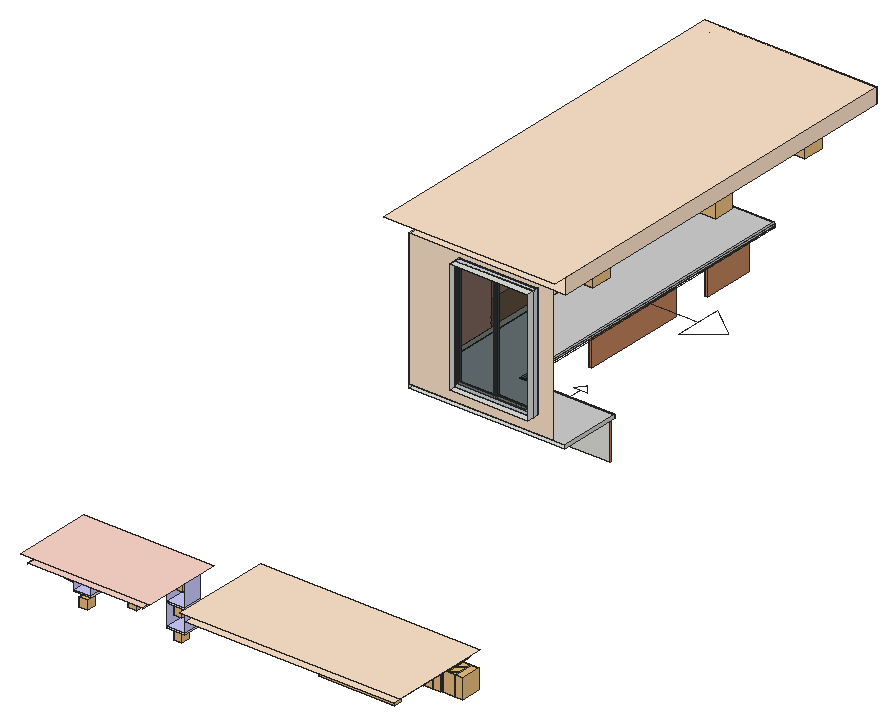
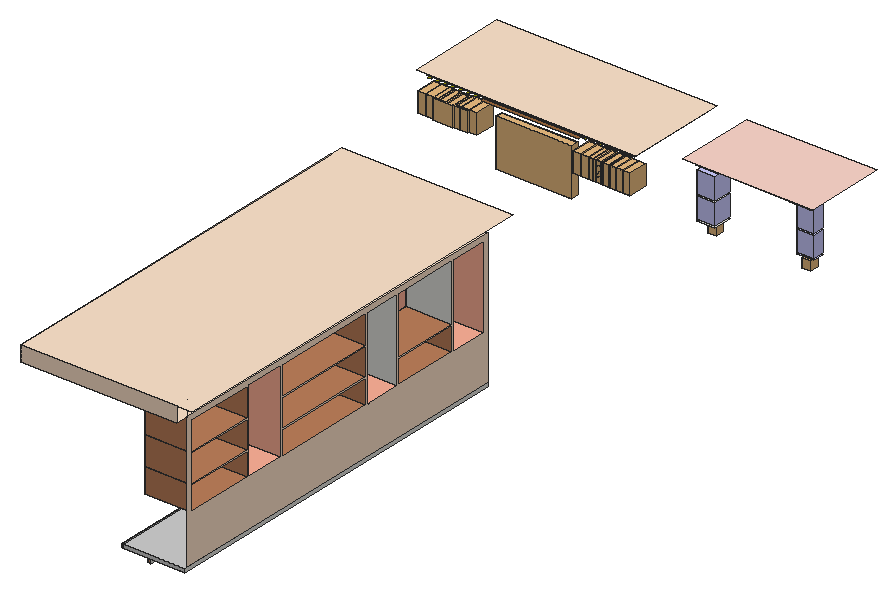
# SketchUp Ruby script. Lengths in inches.
U = 1.inch
M = Sketchup.active_model
def pt(a) = Geom::Point3d.new(a.map { |v| v * U })
def face(e, loops, mat)
  f = e.add_face(loops[0].map { |a| pt(a) })
  loops[1..].each { |l| e.add_face(l.map { |a| pt(a) }).erase! }
  f.material = f.back_material = mat if mat
  f
end
# faces: each face lists its corners as indices into pts; further lists are holes
def faces(e, pts, list, mat = nil) = list.each { |f| face(e, (f[0].is_a?(Array) ? f : [f]).map { |l| l.map { |i| pts[i] } }, mat) }
# xy, xz, yz: faces in a plane at the given z, y or x. An outline is a flat list of corners, or four numbers for a rectangle; further outlines are holes
def ring(l) = l.size == 4 ? [[l[0], l[1]], [l[2], l[1]], [l[2], l[3]], [l[0], l[3]]] : l.each_slice(2).to_a
def flat(e, list, mat, &to3) = list.each { |f| face(e, (f[0].is_a?(Array) ? f : [f]).map { |l| ring(l).map { |u, v| to3.(u, v) } }, mat) }
def xy(e, z, list, mat = nil) = flat(e, list, mat) { |x, y| [x, y, z] }
def xz(e, y, list, mat = nil) = flat(e, list, mat) { |x, z| [x, y, z] }
def yz(e, x, list, mat = nil) = flat(e, list, mat) { |y, z| [x, y, z] }
def lines(e, pts, list) = list.each { |a, b| e.add_line(pt(pts[a]), pt(pts[b])) }
# prism: a flat outline (further loops are holes) pulled along v
def prism(e, loops, v, mat = nil)
  f = face(e, loops, mat); d = Geom::Vector3d.new(v.map { |x| x * U })
  f.pushpull(f.normal.samedirection?(d) ? d.length : -d.length)
end
def box(e, o, s, mat = nil) = prism(e, [[o, [o[0] + s[0], o[1], o[2]], [o[0] + s[0], o[1] + s[1], o[2]], [o[0], o[1] + s[1], o[2]]]], [0, 0, s[2]], mat)
def at(x, y, z, deg = 0) = Geom::Transformation.translation(pt([x, y, z])) * Geom::Transformation.rotation(ORIGIN, Z_AXIS, deg.degrees)
def axes(o, x, y, z) = Geom::Transformation.new([*x, 0, *y, 0, *z, 0, *pt(o).to_a, 1])
def part(name) = M.definitions.add(name)
# library, detail: a bought-in or finely detailed component or shape, given as its bounding box
def library(name, o, s) = part(name).tap { |d| box(d.entities, o, s) }
def detail(e, o, s) = box(e.add_group.entities, o, s)
def put(e, d, t, mat = nil) = e.add_instance(d, t).tap { |i| i.material = mat if mat }
def group(e, t, mat = nil) = e.add_group.tap { |g| g.transformation = t; g.material = mat if mat }.entities
root = M.entities
M.materials.add("[Carrera Marble]").color = [207, 207, 207]
M.materials.add("[Color B01]").color = [255, 216, 204]
M.materials.add("[Color B02]").color = [255, 178, 153]
M.materials.add("[Color C01]").color = [255, 229, 204]
M.materials.add("[Color E07]").color = [153, 153, 0]
M.materials.add("[Color F02]").color = [204, 255, 153]
M.materials.add("[Color I01]").color = [204, 204, 255]
M.materials.add("[Metal Aluminum Anodized]").color = [202, 209, 219]
M.materials.add("[Metal Seamed]").color = [118, 119, 115]
M.materials.add("[Translucent Glass Tinted]").color = [1, 25, 30]
M.materials["[Translucent Glass Tinted]"].alpha = 0.31
M.materials.add("[Wood Floor]").color = [155, 105, 61]
M.materials.add("[Wood Veneer 02]").color = [190, 128, 91]
c1 = library("Spot Light\#1",[-5.1,-5.1,-11.05],[10.2,10.2,11.05])
c2 = library("Flat screen display",[0,1.41,1.14],[35.92,0.28,20.21])
c3 = library("Spot Light\#2",[-5.1,-5.1,-11.05],[10.2,10.2,11.05])
c4 = library("Omni Light",[-12,-12,-12],[24,24,24])
c5 = part("Group33\#1")
p = [[0,0,0],[0,0,-18.23],[-8.72,0,-18.23],[56.77,-2.25,0],[-56.77,-2.25,0],[56.77,2.25,0],
  [56.77,0,0],[-56.77,2.25,0],[8.72,0,-18.23],[-56.77,0,0],[0,0,-29.51]]
lines(c5.entities,p,[[0,1],[1,2],[3,4],[5,6],[7,5],[1,8],[9,0],[0,6],[8,10],[4,9],[6,3],[2,10],
  [9,7]])
c6 = part("Rectangle Light")
put(c6.entities,c5,at(0,0,0))
c7 = part("Group35\#1")
p = [[0,0,0],[0,0,-59.7],[-29.34,0,-59.7],[191.03,-2.25,0],[-191.03,-2.25,0],[191.03,2.25,0],
  [191.03,0,0],[-191.03,2.25,0],[29.34,0,-59.7],[-191.03,0,0],[0,0,-96.64]]
lines(c7.entities,p,[[0,1],[1,2],[3,4],[5,6],[7,5],[1,8],[9,0],[0,6],[8,10],[4,9],[6,3],[2,10],
  [9,7]])
c8 = part("Rectangle Light\#1")
put(c8.entities,c7,at(0,0,0))
c9 = library("Spot Light\#3",[-5.1,-5.1,-11.05],[10.2,10.2,11.05])
c10 = part("Group\#106")
prism(c10.entities,[[[0.375,0,0],[0.375,0,57],[0.375,26.94,57],[0.375,26.94,0]],[[0.375,25.82,55.875],[0.375,1.125,55.875],[0.375,1.125,1.125],[0.375,25.82,1.125]]],[1.5,0,0])
c11 = part("Group\#67")
box(c11.entities,[0,-23.19,0],[1.125,24.69,54.75])
c12 = part("Aluminium+Channel+Glass+Window")
g1 = group(c12.entities,at(536.45,-8.32,338.57,90))
g2 = group(g1,at(73.57,-163.55,-184.94),"[Metal Aluminum Anodized]")
prism(g2,[[[0,0,136.125],[0,94.5,136.125],[0,94.5,0],[0,0,0]],[[0,2.49,3.4],[0,92.01,3.4],[0,92.01,132.72],[0,2.49,132.72]]],[5.375,0,0])
g3 = group(g1,at(76.3,-161.06,-181.54))
put(g3,c10,axes([-0.55,0,0],[1.45782,0,0],[0,1.69662,0],[0,0,2.26875]),"[Metal Seamed]")
put(g3,c11,axes([0.27,41.26,2.55],[1.45782,0,0],[0,1.69662,0],[0,0,2.26875]),"[Translucent Glass Tinted]")
g4 = group(g1,at(74.11,-117.25,-181.54))
put(g4,c10,axes([-0.55,0,0],[1.45782,0,0],[0,1.69662,0],[0,0,2.26875]),"[Metal Seamed]")
put(g4,c11,axes([0.27,41.26,2.55],[1.45782,0,0],[0,1.69662,0],[0,0,2.26875]),"[Translucent Glass Tinted]")
c13 = library("Spot Light",[-5.1,-5.1,-11.05],[10.2,10.2,11.05])
xy(root,81.2,[[164.74,586.56,240.3,588.31]])
xy(root,89.47,[[122.73,67.26,144.4375,90.2]])
xy(root,89.48,[[11.17,67.26,31.62,80.32]],"[Color I01]")
xy(root,91.47,[[122.73,67.26,144.4375,90.2]],"[Color I01]")
xy(root,91.48,[[11.17,67.26,31.62,80.32]],"[Color I01]")
xy(root,96.13,[[126.97,696.29,126.78,823.17,130.96,823.18,131.14,696.3],[126.97,871.55,126.78,932.72,130.58,932.73,130.76,871.56]])
xy(root,116.16,[[122.73,67.26,144.4375,90.2]])
xy(root,116.18,[[11.17,67.26,31.62,80.32]],"[Color I01]")
xy(root,118.16,[[122.73,67.26,144.4375,90.2]],"[Color I01]")
xy(root,118.18,[[11.17,67.26,31.62,80.32]],"[Color I01]")
xy(root,120.1875,[[207.4,109.94,211.04,115.88],[216.41,109.94,220.05,115.88],[225.42,109.94,229.06,115.88],[234.43,109.94,238.08,115.88],[243.44,109.94,247.09,115.88],
  [252.45,109.94,256.1,115.88],[392.64,109.94,396.28,115.88],[401.81,109.94,405.45,115.88],[410.97,109.94,414.62,115.88],[420.14,109.94,423.78,115.88],
  [429.31,109.94,432.95,115.88],[438.47,109.94,442.12,115.88]],"[Color F02]")
xy(root,127.26,[[164.74,586.56,240.3,588.31],[126.97,696.29,131.14,696.3,130.96,823.18,126.78,823.17],[126.97,871.55,130.76,871.56,130.58,932.73,126.78,932.72]],"[Wood Veneer 02]")
xy(root,128.0625,[[55.53,515.38,55.53,971,130.28,971,130.28,588.93,243.82,588.93,243.82,515.38]])
xy(root,132.5625,[[55.53,515.38,243.82,515.38,243.82,588.93,130.28,588.93,130.28,971,55.53,971]],"[Carrera Marble]")
xy(root,144.85,[[122.73,67.26,144.4375,90.2]],"[Color I01]")
xy(root,144.88,[[11.17,67.26,31.62,80.32]],"[Color I01]")
xy(root,147.04,[[264.93,112.26,382.43,115.88]],"[Wood Floor]")
xy(root,147.5625,[[8.49,67.26,34.3,87.7],[120.02,67.26,147.15,87.7]],"[Color I01]")
xy(root,148.5,[[[8.49,0,147.15,87.7],[46.53,12.51,48.28,12.74,49.91,13.41,51.31,14.48,52.38,15.88,53.05,17.51,53.28,19.26,53.05,21,52.38,22.63,51.31,24.03,49.91,25.1,48.28,25.78,46.53,26.01,44.79,25.78,43.16,25.1,41.76,24.03,40.6875,22.63,40.01,21,39.78,19.26,40.01,17.51,40.6875,15.88,41.76,14.48,43.16,13.41,44.79,12.74],[90.51,47.29,91.79,47.46,92.98,47.95,94,48.74,94.79,49.76,95.28,50.95,95.45,52.23,95.28,53.51,94.79,54.7,94,55.72,92.98,56.51,91.79,57,90.51,57.17,89.23,57,88.04,56.51,87.02,55.72,86.23,54.7,85.74,53.51,85.57,52.23,85.74,50.95,86.23,49.76,87.02,48.74,88.04,47.95,89.23,47.46],[126.44,11.29,127.7,11.46,128.88,11.94,129.89,12.72,130.66,13.73,131.15,14.9,131.32,16.17,131.15,17.43,130.66,18.6,129.89,19.61,128.88,20.39,127.7,20.875,126.44,21.04,125.18,20.875,124,20.39,122.99,19.61,122.22,18.6,121.73,17.43,121.57,16.17,121.73,14.9,122.22,13.73,122.99,12.72,124,11.94,125.18,11.46]],[[126.44,11.29,125.18,11.46,124,11.94,122.99,12.72,122.22,13.73,121.73,14.9,121.57,16.17,121.73,17.43,122.22,18.6,122.99,19.61,124,20.39,125.18,20.875,126.44,21.04,127.7,20.875,128.88,20.39,129.89,19.61,130.66,18.6,131.15,17.43,131.32,16.17,131.15,14.9,130.66,13.73,129.89,12.72,128.88,11.94,127.7,11.46],[126.44,12.49,127.39,12.61,128.28,12.98,129.04,13.5625,129.63,14.33,130,15.21,130.12,16.17,130,17.12,129.63,18.01,129.04,18.77,128.28,19.35,127.39,19.72,126.44,19.85,125.49,19.72,124.6,19.35,123.84,18.77,123.25,18.01,122.89,17.12,122.76,16.17,122.89,15.21,123.25,14.33,123.84,13.5625,124.6,12.98,125.49,12.61]],[[46.53,12.51,44.79,12.74,43.16,13.41,41.76,14.48,40.6875,15.88,40.01,17.51,39.78,19.26,40.01,21,40.6875,22.63,41.76,24.03,43.16,25.1,44.79,25.78,46.53,26.01,48.28,25.78,49.91,25.1,51.31,24.03,52.38,22.63,53.05,21,53.28,19.26,53.05,17.51,52.38,15.88,51.31,14.48,49.91,13.41,48.28,12.74],[46.53,15.02,47.63,15.16,48.65,15.59,49.53,16.26,50.2,17.14,50.63,18.16,50.77,19.26,50.63,20.35,50.2,21.375,49.53,22.25,48.65,22.93,47.63,23.35,46.53,23.5,45.4375,23.35,44.41,22.93,43.54,22.25,42.86,21.375,42.44,20.35,42.3,19.26,42.44,18.16,42.86,17.14,43.54,16.26,44.41,15.59,45.4375,15.16]],[[90.51,47.29,89.23,47.46,88.04,47.95,87.02,48.74,86.23,49.76,85.74,50.95,85.57,52.23,85.74,53.51,86.23,54.7,87.02,55.72,88.04,56.51,89.23,57,90.51,57.17,91.79,57,92.98,56.51,94,55.72,94.79,54.7,95.28,53.51,95.45,52.23,95.28,50.95,94.79,49.76,94,48.74,92.98,47.95,91.79,47.46],[90.51,48.76,91.41,48.88,92.24,49.22,92.96,49.78,93.52,50.49,93.86,51.33,93.98,52.23,93.86,53.13,93.52,53.97,92.96,54.68,92.24,55.24,91.41,55.58,90.51,55.7,89.61,55.58,88.77,55.24,88.05,54.68,87.5,53.97,87.16,53.13,87.04,52.23,87.16,51.33,87.5,50.49,88.05,49.78,88.77,49.22,89.61,48.88]]],"[Color B01]")
xy(root,149,[[202.89,109.94,206.54,115.88],[211.9,109.94,215.55,115.88],[220.91,109.94,224.56,115.88],[229.92,109.94,233.57,115.88],[238.94,109.94,242.58,115.88],
  [247.95,109.94,251.59,115.88],[256.96,109.94,260.6,115.88],[388.06,109.94,391.7,115.88],[397.22,109.94,400.87,115.88],[406.39,109.94,410.03,115.88],
  [415.56,109.94,419.2,115.88],[424.72,109.94,428.37,115.88],[433.89,109.94,437.53,115.88],[443.06,109.94,446.7,115.88]],"[Color E07]")
xy(root,149.6875,[[126.44,12.49,125.49,12.61,124.6,12.98,123.84,13.5625,123.25,14.33,122.89,15.21,122.76,16.17,122.89,17.12,123.25,18.01,123.84,18.77,124.6,19.35,125.49,19.72,126.44,19.85,127.39,19.72,128.28,19.35,129.04,18.77,129.63,18.01,130,17.12,130.12,16.17,130,15.21,129.63,14.33,129.04,13.5625,128.28,12.98,127.39,12.61]],"[Color B01]")
xy(root,149.8125,[[46.53,15.02,45.4375,15.16,44.41,15.59,43.54,16.26,42.86,17.14,42.44,18.16,42.3,19.26,42.44,20.35,42.86,21.375,43.54,22.25,44.41,22.93,45.4375,23.35,46.53,23.5,47.63,23.35,48.65,22.93,49.53,22.25,50.2,21.375,50.63,20.35,50.77,19.26,50.63,18.16,50.2,17.14,49.53,16.26,48.65,15.59,47.63,15.16]],"[Color B01]")
xy(root,150.875,[[90.51,48.76,89.61,48.88,88.77,49.22,88.05,49.78,87.5,50.49,87.16,51.33,87.04,52.23,87.16,53.13,87.5,53.97,88.05,54.68,88.77,55.24,89.61,55.58,90.51,55.7,91.41,55.58,92.24,55.24,92.96,54.68,93.52,53.97,93.86,53.13,93.98,52.23,93.86,51.33,93.52,50.49,92.96,49.78,92.24,49.22,91.41,48.88]],"[Color B01]")
xy(root,151.1875,[[197.89,1.64,448.06,115.88]],"[Color C01]")
xy(root,153.625,[[116.72,499.97,211.22,515.38]])
xy(root,155.125,[[0,0,156.26,96.1875]],"[Color B01]")
xy(root,158,[[190.88,1.64,455.07,122.89]],"[Color C01]")
xy(root,189.5,[[55.53,521.38,111.53,568.07],[55.53,651.49,111.53,697.87],[55.53,826.92,111.53,875.98]],"[Color B02]")
xy(root,189.5,[[55.53,568.97,111.53,650.59],[55.53,698.77,111.53,826.02],[55.53,876.88,111.53,961.6875]],"[Wood Veneer 02]")
xy(root,218.3125,[[55.53,568.97,111.53,650.59],[55.53,698.77,111.53,826.02],[55.53,876.88,111.53,961.6875]],"[Wood Veneer 02]")
xy(root,219.11,[[55.53,568.97,111.53,650.59],[55.53,698.77,111.53,826.02],[55.53,876.88,111.53,961.6875]],"[Wood Veneer 02]")
xy(root,252.6875,[[55.53,698.77,111.53,826.02],[55.53,876.88,111.53,961.6875]],"[Wood Veneer 02]")
xy(root,253.59,[[55.53,698.77,111.53,826.02],[55.53,876.88,111.53,961.6875]],"[Wood Veneer 02]")
xy(root,288.5,[[55.53,521.38,111.53,568.07],[55.53,568.97,111.53,650.59],[55.53,651.49,111.53,697.87],[55.53,826.92,111.53,875.98]],"[Color B02]")
xy(root,288.5,[[55.53,698.77,111.53,826.02],[55.53,876.88,111.53,961.6875]],"[Wood Veneer 02]")
xy(root,289.75,[[116.72,499.97,211.22,515.38]])
xy(root,294.5,[[[55.53,515.38,244.12,983.1],[215.11,894.45,218.83,895.12,222.26,896.74,225.15,899.18,227.31,902.29,228.59,905.85,228.9,909.625,228.23,913.35,226.62,916.77,224.17,919.66,221.0625,921.82,217.5,923.1,213.73,923.42,210,922.75,206.58,921.13,203.6875,918.6875,201.53,915.58,200.25,912.02,199.93,908.24,200.61,904.52,202.22,901.1,204.66,898.21,207.77,896.05,211.34,894.77],[210.38,581.74,214.09,582.23,217.54,583.66,220.5,585.93,222.78,588.89,224.21,592.35,224.69,596.05,224.21,599.75,222.78,603.21,220.5,606.17,217.54,608.45,214.09,609.875,210.38,610.36,206.68,609.875,203.23,608.45,200.26,606.17,197.99,603.21,196.56,599.75,196.07,596.05,196.56,592.35,197.99,588.89,200.26,585.93,203.23,583.66,206.68,582.23],[216.58,753.94,220.08,754.58,223.29,756.1,226.01,758.39,228.03,761.32,229.23,764.67,229.52,768.21,228.89,771.71,227.37,774.93,225.07,777.64,222.15,779.67,218.8,780.87,215.26,781.16,211.76,780.53,208.54,779.01,205.83,776.71,203.8,773.78,202.6,770.4375,202.31,766.89,202.94,763.39,204.46,760.18,206.76,757.46,209.68,755.44,213.03,754.23]],[[210.38,581.74,206.68,582.23,203.23,583.66,200.26,585.93,197.99,588.89,196.56,592.35,196.07,596.05,196.56,599.75,197.99,603.21,200.26,606.17,203.23,608.45,206.68,609.875,210.38,610.36,214.09,609.875,217.54,608.45,220.5,606.17,222.78,603.21,224.21,599.75,224.69,596.05,224.21,592.35,222.78,588.89,220.5,585.93,217.54,583.66,214.09,582.23],[210.15,583.74,213.35,584.1,216.34,585.27,218.92,587.18,220.93,589.7,222.21,592.64,222.69,595.82,222.33,599.01,221.16,602.01,219.25,604.59,216.74,606.6,213.79,607.88,210.61,608.36,207.42,608,204.43,606.83,201.84,604.92,199.84,602.41,198.55,599.46,198.07,596.28,198.43,593.09,199.61,590.09,201.51,587.51,204.03,585.5,206.97,584.22]],[[216.58,753.94,213.03,754.23,209.68,755.44,206.76,757.46,204.46,760.18,202.94,763.39,202.31,766.89,202.6,770.4375,203.8,773.78,205.83,776.71,208.54,779.01,211.76,780.53,215.26,781.16,218.8,780.87,222.15,779.67,225.07,777.64,227.37,774.93,228.89,771.71,229.52,768.21,229.23,764.67,228.03,761.32,226.01,758.39,223.29,756.1,220.08,754.58],[214.42,756.02,217.46,756.03,220.39,756.82,223.01,758.34,225.15,760.49,226.67,763.125,227.44,766.06,227.4375,769.09,226.65,772.02,225.125,774.65,222.97,776.79,220.34,778.3,217.41,779.08,214.375,779.07,211.44,778.28,208.82,776.76,206.68,774.61,205.17,771.98,204.39,769.04,204.39,766.01,205.19,763.08,206.71,760.45,208.86,758.3125,211.49,756.8]],[[215.11,894.45,211.34,894.77,207.77,896.05,204.66,898.21,202.22,901.1,200.61,904.52,199.93,908.24,200.25,912.02,201.53,915.58,203.6875,918.6875,206.58,921.13,210,922.75,213.73,923.42,217.5,923.1,221.0625,921.82,224.17,919.66,226.62,916.77,228.23,913.35,228.9,909.625,228.59,905.85,227.31,902.29,225.15,899.18,222.26,896.74,218.83,895.12],[214.42,896.85,217.55,897.26,220.46,898.47,222.96,900.39,224.88,902.89,226.09,905.81,226.5,908.93,226.09,912.0625,224.88,914.98,222.96,917.48,220.46,919.4,217.55,920.61,214.42,921.02,211.29,920.61,208.375,919.4,205.87,917.48,203.95,914.98,202.74,912.0625,202.33,908.93,202.74,905.81,203.95,902.89,205.87,900.39,208.375,898.47,211.29,897.26]]],"[Color C01]")
xy(root,296.75,[[214.42,756.02,211.49,756.8,208.86,758.3125,206.71,760.45,205.19,763.08,204.39,766.01,204.39,769.04,205.17,771.98,206.68,774.61,208.82,776.76,211.44,778.28,214.375,779.07,217.41,779.08,220.34,778.3,222.97,776.79,225.125,774.65,226.65,772.02,227.4375,769.09,227.44,766.06,226.67,763.125,225.15,760.49,223.01,758.34,220.39,756.82,217.46,756.03]],"[Color C01]")
xy(root,297.3125,[[210.15,583.74,206.97,584.22,204.03,585.5,201.51,587.51,199.61,590.09,198.43,593.09,198.07,596.28,198.55,599.46,199.84,602.41,201.84,604.92,204.43,606.83,207.42,608,210.61,608.36,213.79,607.88,216.74,606.6,219.25,604.59,221.16,602.01,222.33,599.01,222.69,595.82,222.21,592.64,220.93,589.7,218.92,587.18,216.34,585.27,213.35,584.1]],"[Color C01]")
xy(root,297.4375,[[214.42,896.85,211.29,897.26,208.375,898.47,205.87,900.39,203.95,902.89,202.74,905.81,202.33,908.93,202.74,912.0625,203.95,914.98,205.87,917.48,208.375,919.4,211.29,920.61,214.42,921.02,217.55,920.61,220.46,919.4,222.96,917.48,224.88,914.98,226.09,912.0625,226.5,908.93,226.09,905.81,224.88,902.89,222.96,900.39,220.46,898.47,217.55,897.26]],"[Color C01]")
xy(root,313,[[38.18,499.97,244.12,983.1]],"[Color C01]")
xz(root,80.32,[[11.17,91.48,31.62,116.18],[11.17,118.18,31.62,144.88]],"[Color I01]")
xz(root,87.7,[[8.49,147.5625,34.3,148.5],[120.02,147.5625,147.15,148.5]],"[Color B01]")
xz(root,90.2,[[122.73,91.47,144.4375,116.16],[122.73,118.16,144.4375,144.85]],"[Color I01]")
xz(root,515.38,[[[55.53,132.5625,228.71,294.5],[116.72,153.625,211.22,289.75]]],"[Color C01]")
xz(root,521.38,[[55.53,189.5,111.53,288.5]],"[Color B02]")
xz(root,568.07,[[55.53,189.5,111.53,288.5]],"[Color B02]")
xz(root,568.97,[[55.53,219.11,111.53,288.5]])
xz(root,568.97,[[55.53,189.5,111.53,218.3125]],"[Wood Veneer 02]")
xz(root,586.56,[[164.74,81.2,240.3,127.26]])
xz(root,588.31,[[164.74,81.2,240.3,127.26]],"[Wood Veneer 02]")
xz(root,588.93,[[130.28,128.0625,243.82,132.5625]],"[Carrera Marble]")
xz(root,650.59,[[55.53,219.11,111.53,288.5]],"[Color B02]")
xz(root,650.59,[[55.53,189.5,111.53,218.3125]],"[Wood Veneer 02]")
xz(root,651.49,[[55.53,189.5,111.53,288.5]])
xz(root,697.87,[[55.53,189.5,111.53,288.5]],"[Color B02]")
xz(root,698.77,[[55.53,189.5,111.53,218.3125],[55.53,219.11,111.53,252.6875],[55.53,253.59,111.53,288.5]],"[Wood Veneer 02]")
xz(root,826.02,[[55.53,189.5,111.53,218.3125],[55.53,219.11,111.53,252.6875],[55.53,253.59,111.53,288.5]],"[Wood Veneer 02]")
xz(root,826.92,[[55.53,189.5,111.53,288.5]],"[Color B02]")
xz(root,875.98,[[55.53,189.5,111.53,288.5]],"[Color B02]")
xz(root,876.88,[[55.53,189.5,111.53,218.3125],[55.53,219.11,111.53,252.6875],[55.53,253.59,111.53,288.5]],"[Wood Veneer 02]")
xz(root,961.6875,[[55.53,189.5,111.53,218.3125],[55.53,219.11,111.53,252.6875],[55.53,253.59,111.53,288.5]],"[Wood Veneer 02]")
xz(root,971,[[55.53,128.0625,130.28,132.5625]],"[Carrera Marble]")
xz(root,983.1,[[55.53,294.5,244.12,313]],"[Color C01]")
yz(root,8.49,[[0,147.5625,87.7,148.5]],"[Color B01]")
yz(root,11.17,[[67.26,91.48,80.32,116.18],[67.26,118.18,80.32,144.88]],"[Color I01]")
yz(root,31.62,[[67.26,89.48,80.32,91.48],[67.26,116.18,80.32,118.18]])
yz(root,31.62,[[67.26,91.48,80.32,116.18],[67.26,118.18,80.32,144.88]],"[Color I01]")
yz(root,55.53,[[515.38,128.0625,971,132.5625]])
yz(root,55.53,[[[515.38,132.5625,967.6875,294.5],[568.97,219.11,650.59,288.5],[826.92,189.5,875.98,288.5],[521.38,189.5,568.07,288.5],[651.49,189.5,697.87,288.5],[698.77,253.59,826.02,288.5],[698.77,219.11,826.02,252.6875],[698.77,189.5,826.02,218.3125],[876.88,253.59,961.6875,288.5],[876.88,219.11,961.6875,252.6875],[876.88,189.5,961.6875,218.3125],[568.97,189.5,650.59,218.3125]]],"[Color C01]")
yz(root,111.53,[[521.38,189.5,568.07,288.5],[651.49,189.5,697.87,288.5],[826.92,189.5,875.98,288.5],[568.97,219.11,650.59,288.5]],"[Color B02]")
yz(root,111.53,[[568.97,189.5,650.59,218.3125],[698.77,189.5,826.02,218.3125],[876.88,189.5,961.6875,218.3125],[698.77,219.11,826.02,252.6875],[876.88,219.11,961.6875,252.6875],
  [698.77,253.59,826.02,288.5],[876.88,253.59,961.6875,288.5]],"[Wood Veneer 02]")
yz(root,116.72,[[499.97,153.625,515.38,289.75]])
yz(root,122.73,[[67.26,91.47,90.2,116.16],[67.26,118.16,90.2,144.85]],"[Color I01]")
yz(root,130.28,[[588.93,128.0625,971,132.5625]],"[Carrera Marble]")
yz(root,144.4375,[[67.26,89.47,90.2,91.47],[67.26,116.16,90.2,118.16]])
yz(root,144.4375,[[67.26,91.47,90.2,116.16],[67.26,118.16,90.2,144.85]],"[Color I01]")
yz(root,147.15,[[0,147.5625,87.7,148.5]],"[Color B01]")
yz(root,164.74,[[586.56,81.2,588.31,127.26]])
yz(root,204.39,[[766.01,294.5,769.04,296.75]],"[Color C01]")
yz(root,211.22,[[499.97,153.625,515.38,289.75]])
yz(root,240.3,[[586.56,81.2,588.31,127.26]],"[Wood Veneer 02]")
yz(root,243.82,[[515.38,128.0625,588.93,132.5625]],"[Carrera Marble]")
yz(root,244.12,[[515.38,294.5,983.1,313]],"[Color C01]")
p = [[126.97,696.29,96.13],[126.97,696.29,127.26],[126.78,823.17,127.26],[126.78,823.17,96.13],[131.14,696.3,96.13],[131.14,696.3,127.26],
  [130.96,823.18,96.13],[130.96,823.18,127.26],[126.97,871.55,96.13],[126.97,871.55,127.26],[126.78,932.72,127.26],[126.78,932.72,96.13],
  [130.76,871.56,96.13],[130.76,871.56,127.26],[130.58,932.73,96.13],[130.58,932.73,127.26],[126.44,12.49,148.5],[125.49,12.61,148.5],
  [125.49,12.61,149.6875],[126.44,12.49,149.6875],[127.39,12.61,148.5],[127.39,12.61,149.6875],[124.6,12.98,148.5],[124.6,12.98,149.6875],
  [128.28,12.98,148.5],[128.28,12.98,149.6875],[123.84,13.5625,148.5],[123.84,13.5625,149.6875],[129.04,13.5625,148.5],[129.04,13.5625,149.6875],
  [123.25,14.33,148.5],[123.25,14.33,149.6875],[129.63,14.33,148.5],[129.63,14.33,149.6875],[122.89,15.21,148.5],[122.89,15.21,149.6875],
  [130,15.21,148.5],[130,15.21,149.6875],[46.53,15.02,148.5],[45.4375,15.16,148.5],[45.4375,15.16,149.8125],[46.53,15.02,149.8125],
  [47.63,15.16,148.5],[47.63,15.16,149.8125],[44.41,15.59,148.5],[44.41,15.59,149.8125],[48.65,15.59,148.5],[48.65,15.59,149.8125],
  [122.76,16.17,148.5],[122.76,16.17,149.6875],[130.12,16.17,148.5],[130.12,16.17,149.6875],[43.54,16.26,148.5],[43.54,16.26,149.8125],
  [49.53,16.26,148.5],[49.53,16.26,149.8125],[122.89,17.12,148.5],[122.89,17.12,149.6875],[130,17.12,148.5],[130,17.12,149.6875],
  [42.86,17.14,148.5],[42.86,17.14,149.8125],[50.2,17.14,148.5],[50.2,17.14,149.8125],[42.44,18.16,148.5],[42.44,18.16,149.8125],
  [50.63,18.16,148.5],[50.63,18.16,149.8125],[123.25,18.01,148.5],[123.25,18.01,149.6875],[129.63,18.01,148.5],[129.63,18.01,149.6875],
  [123.84,18.77,148.5],[123.84,18.77,149.6875],[129.04,18.77,148.5],[129.04,18.77,149.6875],[42.3,19.26,148.5],[42.3,19.26,149.8125],
  [50.77,19.26,148.5],[50.77,19.26,149.8125],[124.6,19.35,148.5],[124.6,19.35,149.6875],[128.28,19.35,148.5],[128.28,19.35,149.6875],
  [42.44,20.35,148.5],[42.44,20.35,149.8125],[50.63,20.35,148.5],[50.63,20.35,149.8125],[125.49,19.72,148.5],[125.49,19.72,149.6875],
  [127.39,19.72,148.5],[127.39,19.72,149.6875],[126.44,19.85,148.5],[126.44,19.85,149.6875],[42.86,21.375,148.5],[42.86,21.375,149.8125],
  [50.2,21.375,148.5],[50.2,21.375,149.8125],[43.54,22.25,148.5],[43.54,22.25,149.8125],[49.53,22.25,148.5],[49.53,22.25,149.8125],
  [44.41,22.93,148.5],[44.41,22.93,149.8125],[48.65,22.93,148.5],[48.65,22.93,149.8125],[45.4375,23.35,148.5],[45.4375,23.35,149.8125],
  [47.63,23.35,148.5],[47.63,23.35,149.8125],[46.53,23.5,148.5],[46.53,23.5,149.8125],[90.51,48.76,148.5],[89.61,48.88,148.5],
  [89.61,48.88,150.875],[90.51,48.76,150.875],[91.41,48.88,148.5],[91.41,48.88,150.875],[88.77,49.22,148.5],[88.77,49.22,150.875],
  [92.24,49.22,148.5],[92.24,49.22,150.875],[88.05,49.78,148.5],[88.05,49.78,150.875],[92.96,49.78,148.5],[92.96,49.78,150.875],
  [87.5,50.49,148.5],[87.5,50.49,150.875],[93.52,50.49,148.5],[93.52,50.49,150.875],[87.16,51.33,148.5],[87.16,51.33,150.875],
  [93.86,51.33,148.5],[93.86,51.33,150.875],[87.04,52.23,148.5],[87.04,52.23,150.875],[93.98,52.23,148.5],[93.98,52.23,150.875],
  [87.16,53.13,148.5],[87.16,53.13,150.875],[93.86,53.13,148.5],[93.86,53.13,150.875],[87.5,53.97,148.5],[87.5,53.97,150.875],
  [93.52,53.97,148.5],[93.52,53.97,150.875],[88.05,54.68,148.5],[88.05,54.68,150.875],[92.96,54.68,148.5],[92.96,54.68,150.875],
  [88.77,55.24,148.5],[88.77,55.24,150.875],[92.24,55.24,148.5],[92.24,55.24,150.875],[89.61,55.58,148.5],[89.61,55.58,150.875],
  [91.41,55.58,148.5],[91.41,55.58,150.875],[90.51,55.7,148.5],[90.51,55.7,150.875],[210.15,583.74,294.5],[206.97,584.22,294.5],
  [206.97,584.22,297.3125],[210.15,583.74,297.3125],[213.35,584.1,294.5],[213.35,584.1,297.3125],[216.34,585.27,294.5],[216.34,585.27,297.3125],
  [204.03,585.5,294.5],[204.03,585.5,297.3125],[218.92,587.18,294.5],[218.92,587.18,297.3125],[201.51,587.51,294.5],[201.51,587.51,297.3125],
  [220.93,589.7,294.5],[220.93,589.7,297.3125],[199.61,590.09,294.5],[199.61,590.09,297.3125],[222.21,592.64,294.5],[222.21,592.64,297.3125],
  [198.43,593.09,294.5],[198.43,593.09,297.3125],[222.69,595.82,294.5],[222.69,595.82,297.3125],[198.07,596.28,294.5],[198.07,596.28,297.3125],
  [222.33,599.01,294.5],[222.33,599.01,297.3125],[198.55,599.46,294.5],[198.55,599.46,297.3125],[221.16,602.01,294.5],[221.16,602.01,297.3125],
  [199.84,602.41,294.5],[199.84,602.41,297.3125],[219.25,604.59,294.5],[219.25,604.59,297.3125],[201.84,604.92,294.5],[201.84,604.92,297.3125],
  [216.74,606.6,294.5],[216.74,606.6,297.3125],[204.43,606.83,294.5],[204.43,606.83,297.3125],[213.79,607.88,294.5],[213.79,607.88,297.3125],
  [207.42,608,294.5],[207.42,608,297.3125],[210.61,608.36,294.5],[210.61,608.36,297.3125],[214.42,756.02,294.5],[211.49,756.8,294.5],
  [211.49,756.8,296.75],[214.42,756.02,296.75],[217.46,756.03,294.5],[217.46,756.03,296.75],[220.39,756.82,294.5],[220.39,756.82,296.75],
  [208.86,758.3125,294.5],[208.86,758.3125,296.75],[223.01,758.34,294.5],[223.01,758.34,296.75],[206.71,760.45,294.5],[206.71,760.45,296.75],
  [225.15,760.49,294.5],[225.15,760.49,296.75],[205.19,763.08,294.5],[205.19,763.08,296.75],[226.67,763.125,294.5],[226.67,763.125,296.75],
  [204.39,766.01,294.5],[204.39,766.01,296.75],[227.44,766.06,294.5],[227.44,766.06,296.75],[227.4375,769.09,294.5],[227.4375,769.09,296.75],
  [204.39,769.04,294.5],[205.17,771.98,294.5],[205.17,771.98,296.75],[204.39,769.04,296.75],[226.65,772.02,294.5],[226.65,772.02,296.75],
  [206.68,774.61,294.5],[206.68,774.61,296.75],[225.125,774.65,294.5],[225.125,774.65,296.75],[208.82,776.76,294.5],[208.82,776.76,296.75],
  [222.97,776.79,294.5],[222.97,776.79,296.75],[211.44,778.28,294.5],[211.44,778.28,296.75],[220.34,778.3,294.5],[220.34,778.3,296.75],
  [214.375,779.07,294.5],[214.375,779.07,296.75],[217.41,779.08,294.5],[217.41,779.08,296.75],[214.42,896.85,294.5],[211.29,897.26,294.5],
  [211.29,897.26,297.4375],[214.42,896.85,297.4375],[217.55,897.26,294.5],[217.55,897.26,297.4375],[208.375,898.47,294.5],[208.375,898.47,297.4375],
  [220.46,898.47,294.5],[220.46,898.47,297.4375],[205.87,900.39,294.5],[205.87,900.39,297.4375],[222.96,900.39,294.5],[222.96,900.39,297.4375],
  [203.95,902.89,294.5],[203.95,902.89,297.4375],[224.88,902.89,294.5],[224.88,902.89,297.4375],[202.74,905.81,294.5],[202.74,905.81,297.4375],
  [226.09,905.81,294.5],[226.09,905.81,297.4375],[202.33,908.93,294.5],[202.33,908.93,297.4375],[226.5,908.93,294.5],[226.5,908.93,297.4375],
  [202.74,912.0625,294.5],[202.74,912.0625,297.4375],[226.09,912.0625,294.5],[226.09,912.0625,297.4375],[203.95,914.98,294.5],[203.95,914.98,297.4375],
  [224.88,914.98,294.5],[224.88,914.98,297.4375],[205.87,917.48,294.5],[205.87,917.48,297.4375],[222.96,917.48,294.5],[222.96,917.48,297.4375],
  [208.375,919.4,294.5],[208.375,919.4,297.4375],[220.46,919.4,294.5],[220.46,919.4,297.4375],[211.29,920.61,294.5],[211.29,920.61,297.4375],
  [217.55,920.61,294.5],[217.55,920.61,297.4375],[214.42,921.02,294.5],[214.42,921.02,297.4375],[55.53,967.6875,294.5],[55.53,967.6875,313]]
faces(root,p,[[0,1,2,3],[8,9,10,11]])
faces(root,p,[[1,0,4,5],[5,4,6,7],[9,8,12,13],[13,12,14,15],[11,10,15,14]],"[Wood Veneer 02]")
faces(root,p,[[3,2,7,6]],"[Color B02]")
faces(root,p,[[16,17,18,19],[20,16,19,21],[17,22,23,18],[24,20,21,25],[22,26,27,23],[28,24,25,29],[26,30,31,27],[32,28,29,33],
  [30,34,35,31],[36,32,33,37],[38,39,40,41],[42,38,41,43],[39,44,45,40],[46,42,43,47],[34,48,49,35],[50,36,37,51],
  [44,52,53,45],[54,46,47,55],[48,56,57,49],[58,50,51,59],[52,60,61,53],[62,54,55,63],[60,64,65,61],[66,62,63,67],
  [56,68,69,57],[70,58,59,71],[68,72,73,69],[74,70,71,75],[64,76,77,65],[78,66,67,79],[72,80,81,73],[82,74,75,83],
  [76,84,85,77],[86,78,79,87],[80,88,89,81],[90,82,83,91],[88,92,93,89],[92,90,91,93],[84,94,95,85],[96,86,87,97],
  [94,98,99,95],[100,96,97,101],[98,102,103,99],[104,100,101,105],[102,106,107,103],[108,104,105,109],[106,110,111,107],[110,108,109,111],
  [112,113,114,115],[116,112,115,117],[113,118,119,114],[120,116,117,121],[118,122,123,119],[124,120,121,125],[122,126,127,123],[128,124,125,129],
  [126,130,131,127],[132,128,129,133],[130,134,135,131],[136,132,133,137],[134,138,139,135],[140,136,137,141],[138,142,143,139],[144,140,141,145],
  [142,146,147,143],[148,144,145,149],[146,150,151,147],[152,148,149,153],[150,154,155,151],[156,152,153,157],[154,158,159,155],[158,156,157,159]],"[Color B01]")
faces(root,p,[[160,161,162,163],[164,160,163,165],[166,164,165,167],[161,168,169,162],[170,166,167,171],[168,172,173,169],[174,170,171,175],[172,176,177,173],
  [178,174,175,179],[176,180,181,177],[182,178,179,183],[180,184,185,181],[186,182,183,187],[184,188,189,185],[190,186,187,191],[188,192,193,189],
  [194,190,191,195],[192,196,197,193],[198,194,195,199],[196,200,201,197],[202,198,199,203],[200,204,205,201],[206,202,203,207],[204,206,207,205],
  [208,209,210,211],[212,208,211,213],[214,212,213,215],[209,216,217,210],[218,214,215,219],[216,220,221,217],[222,218,219,223],[220,224,225,221],
  [226,222,223,227],[224,228,229,225],[230,226,227,231],[232,230,231,233],[234,235,236,237],[238,232,233,239],[235,240,241,236],[242,238,239,243],
  [240,244,245,241],[246,242,243,247],[244,248,249,245],[250,246,247,251],[248,252,253,249],[254,250,251,255],[252,254,255,253],[256,257,258,259],
  [260,256,259,261],[257,262,263,258],[264,260,261,265],[262,266,267,263],[268,264,265,269],[266,270,271,267],[272,268,269,273],[270,274,275,271],
  [276,272,273,277],[274,278,279,275],[280,276,277,281],[278,282,283,279],[284,280,281,285],[282,286,287,283],[288,284,285,289],[286,290,291,287],
  [292,288,289,293],[290,294,295,291],[296,292,293,297],[294,298,299,295],[300,296,297,301],[298,302,303,299],[302,300,301,303]],"[Color C01]")
lines(root,p,[[304,305]])
put(root,c1,at(22.06,72.69,85.49))
put(root,c2,axes([277.49,61.6,72.7],[2.53506,0,0],[0,29.39676,0],[0,0,2.83082]))
put(root,c3,at(131.8,77.15,87.1))
put(root,c1,at(22.06,72.69,111.61))
put(root,c3,at(131.8,77.15,113.79))
put(root,c4,at(413.58,112.32,124.45))
put(root,c4,at(421.625,113.75,124.45))
put(root,c4,at(209.97,110.91,124.45))
put(root,c4,at(218.79,110.91,124.45))
put(root,c4,at(226.91,110.91,124.45))
put(root,c4,at(236.04,110.91,124.45))
put(root,c4,at(244.91,110.91,124.45))
put(root,c4,at(254.85,110.91,124.45))
put(root,c4,at(394.66,110.91,124.45))
put(root,c4,at(404.08,112.32,124.45))
put(root,c4,at(431.38,112.34,124.75))
put(root,c4,at(440.45,112.34,124.75))
put(root,c6,axes([187.05,590.63,130.3125],[-1,0,0],[0,0,-1],[0,-1,0]))
put(root,c8,axes([132.35,779.97,130.3125],[0,1,0],[0,0,-1],[-1,0,0]))
put(root,c3,at(133.18,77.13,142.35))
put(root,c1,at(22.06,72.69,142.87))
put(root,c9,at(126.47,15.68,147))
put(root,c9,at(90.51,52.23,148.5))
put(root,c9,at(46.61,19.49,148.5625))
put(root,c12,at(-488.78,443.07,0))
put(root,c13,axes([209.34,596.71,291.25],[2.45745,0,0],[0,2.45745,0],[0,0,2.45745]))
put(root,c13,axes([219.26,769.12,292.75],[2.45745,0,0],[0,2.45745,0],[0,0,2.45745]))
put(root,c13,axes([215.27,908.93,294.75],[2.45745,0,0],[0,2.45745,0],[0,0,2.45745]))
